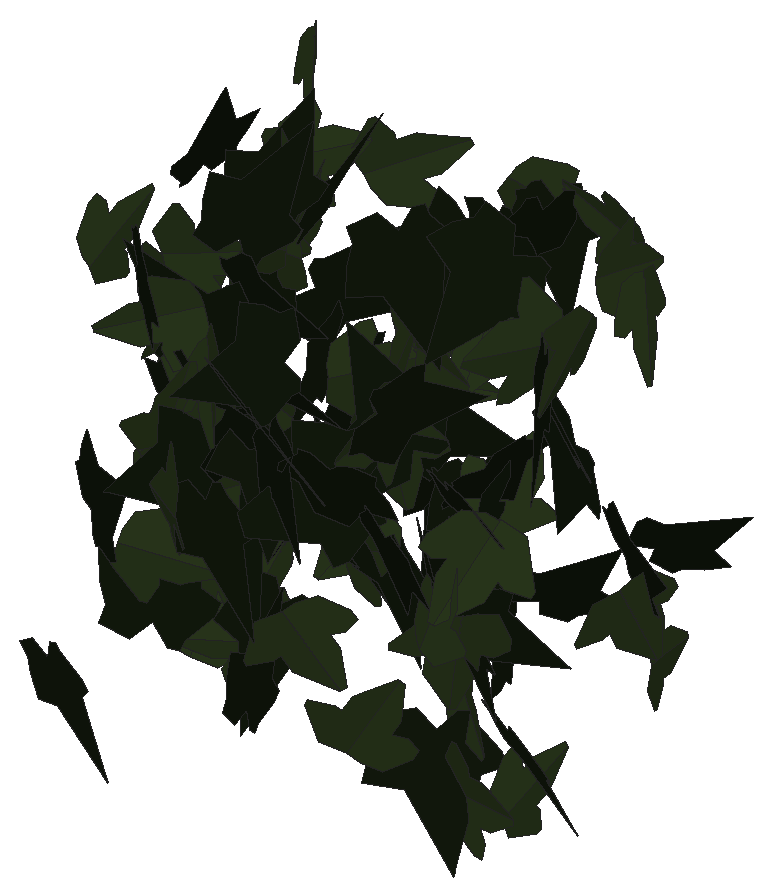
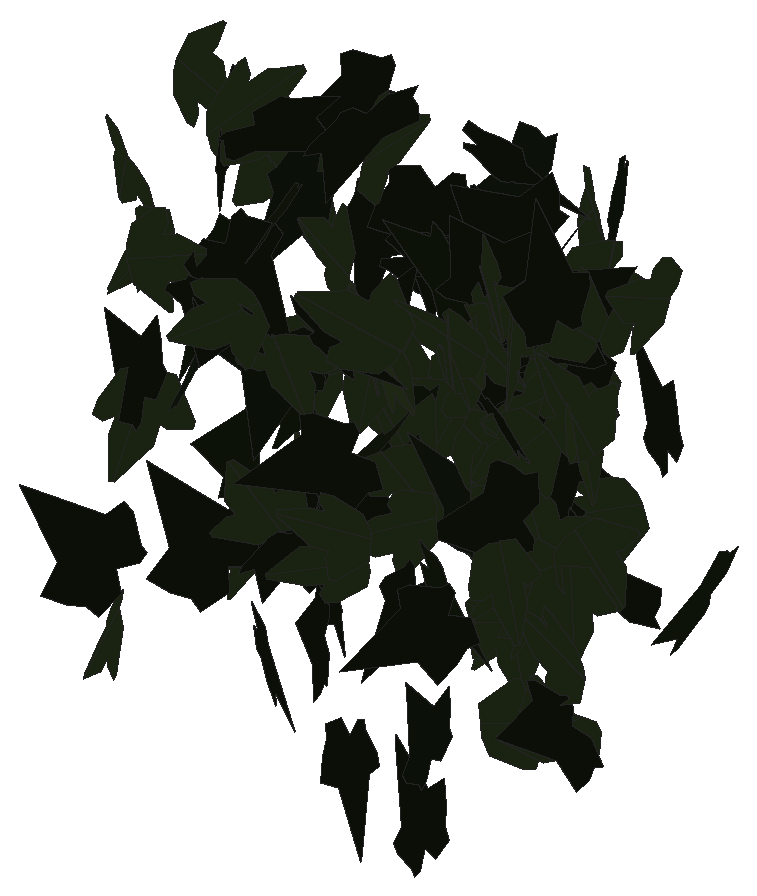
# SketchUp Ruby script. Lengths in inches.
U = 1.inch
M = Sketchup.active_model
def pt(a) = Geom::Point3d.new(a.map { |v| v * U })
def face(e, loops, mat)
  f = e.add_face(loops[0].map { |a| pt(a) })
  loops[1..].each { |l| e.add_face(l.map { |a| pt(a) }).erase! }
  f.material = f.back_material = mat if mat
  f
end
# faces: each face lists its corners as indices into pts; further lists are holes
def faces(e, pts, list, mat = nil) = list.each { |f| face(e, (f[0].is_a?(Array) ? f : [f]).map { |l| l.map { |i| pts[i] } }, mat) }
# xy, xz, yz: faces in a plane at the given z, y or x. An outline is a flat list of corners, or four numbers for a rectangle; further outlines are holes
def ring(l) = l.size == 4 ? [[l[0], l[1]], [l[2], l[1]], [l[2], l[3]], [l[0], l[3]]] : l.each_slice(2).to_a
def flat(e, list, mat, &to3) = list.each { |f| face(e, (f[0].is_a?(Array) ? f : [f]).map { |l| ring(l).map { |u, v| to3.(u, v) } }, mat) }
def xy(e, z, list, mat = nil) = flat(e, list, mat) { |x, y| [x, y, z] }
def xz(e, y, list, mat = nil) = flat(e, list, mat) { |x, z| [x, y, z] }
def yz(e, x, list, mat = nil) = flat(e, list, mat) { |y, z| [x, y, z] }
def lines(e, pts, list) = list.each { |a, b| e.add_line(pt(pts[a]), pt(pts[b])) }
# prism: a flat outline (further loops are holes) pulled along v
def prism(e, loops, v, mat = nil)
  f = face(e, loops, mat); d = Geom::Vector3d.new(v.map { |x| x * U })
  f.pushpull(f.normal.samedirection?(d) ? d.length : -d.length)
end
def box(e, o, s, mat = nil) = prism(e, [[o, [o[0] + s[0], o[1], o[2]], [o[0] + s[0], o[1] + s[1], o[2]], [o[0], o[1] + s[1], o[2]]]], [0, 0, s[2]], mat)
def at(x, y, z, deg = 0) = Geom::Transformation.translation(pt([x, y, z])) * Geom::Transformation.rotation(ORIGIN, Z_AXIS, deg.degrees)
def axes(o, x, y, z) = Geom::Transformation.new([*x, 0, *y, 0, *z, 0, *pt(o).to_a, 1])
def part(name) = M.definitions.add(name)
# library, detail: a bought-in or finely detailed component or shape, given as its bounding box
def library(name, o, s) = part(name).tap { |d| box(d.entities, o, s) }
def detail(e, o, s) = box(e.add_group.entities, o, s)
def put(e, d, t, mat = nil) = e.add_instance(d, t).tap { |i| i.material = mat if mat }
def group(e, t, mat = nil) = e.add_group.tap { |g| g.transformation = t; g.material = mat if mat }.entities
root = M.entities
M.materials.add("efeu1").color = [18, 25, 13]
M.materials.add("efeu2").color = [43, 57, 29]
c1 = part("ivyleaf_10")
p = [[0,0.5,-0.03],[-0.0625,2.02,-0.43],[-0.19,2.01,-0.46],[-0.54,1.05,-0.29],[-0.52,0.625,-0.18],[-0.83,0.76,-0.28],
  [-1.16,0.64,-0.33],[-1.15,0.33,-0.24],[-0.77,-0.39,0.02],[-0.3,-0.51,0.16],[0.04,-0.48,0.23],[-0.02,2.01,-0.4375],
  [-0.06,2.01,-0.43],[0.04,-0.49,0.23],[0.67,-0.49,0.14],[1.38,0.36,-0.2],[1.375,0.51,-0.24],[0.81,0.65,-0.19],
  [0.62,0.59,-0.15],[0.6,1.09,-0.28],[0.5,1.23,-0.31]]
faces(c1.entities,p,[[0,1,2,3,4,5,6,7,8,9,10],[11,12,0,13,14,15,16,17,18,19,20]],"efeu2")
c2 = part("ivyleaf_9")
p = [[1.54,2.16,1.25],[1.36,2.04,1.19],[-0.21,0.99,0.68],[-0.71,1.11,0.82],[-0.85,0.86,0.67],[-0.8,0.17,0.21],
  [-0.9,-0.01,0.1],[-0.67,-0.16,-0.02],[-0.08,-0.08,-0.05],[-0.03,-0.6,-0.4],[0.65,-0.88,-0.66],[0.83,-0.6,-0.49],
  [1.29,-0.42,-0.43],[1.8125,-0.07,-0.26],[1.21,0.44,0.15]]
faces(c2.entities,p,[[0,1,2,3,4,5,6,7,8,9,10,11,12,13,14]],"efeu1")
put(root,c1,axes([553.45,132.17,176.14],[-0.85734,-0.16884,0.1956],[-0.1875,-0.05992,-0.87353],[0.1778,-0.87732,0.02202]))
put(root,c1,axes([553.49,131.52,176.86],[-0.37338,-0.63209,0.40984],[-0.21331,-0.34998,-0.73412],[0.7225,-0.42999,-0.00494]))
put(root,c2,axes([553,137.13,177.71],[0.13734,0.14282,-0.8781],[-0.03731,0.88864,0.1387],[0.88885,0.01524,0.1415]))
put(root,c1,axes([553.22,129.19,182.25],[0.09536,0.36128,-0.85355],[0.25793,0.81382,0.37328],[0.89025,-0.27448,-0.01672]))
put(root,c2,axes([552.78,132.96,173.17],[0.0399,-0.18792,-0.90793],[0.81902,0.43308,-0.05365],[0.43457,-0.79897,0.18446]))
put(root,c1,axes([553.1,136.66,184.01],[0.52637,-0.38449,0.56942],[0.48204,-0.3045,-0.6512],[0.48961,0.71315,0.02895]))
put(root,c1,axes([552.74,133.1,174.82],[0.16897,-0.13445,-1.04144],[0.90074,-0.52365,0.21374],[-0.53977,-0.91594,0.03067]))
put(root,c1,axes([553.95,133.93,177.36],[-0.78131,0.01087,0.45029],[-0.45023,0.0071,-0.78139],[-0.01296,-0.90175,-0.00072]))
put(root,c1,axes([553.77,131.29,180.03],[0.19835,-0.98061,-0.08831],[-0.01984,0.08609,-1.00046],[0.98438,0.19933,-0.00237]))
put(root,c1,axes([553.29,131.76,179.94],[-0.70315,-0.10498,0.70648],[0.69807,0.10878,0.71094],[-0.15114,0.99081,-0.0032]))
put(root,c2,axes([553.57,132.45,183.16],[0.34971,0.64701,0.51065],[-0.25314,-0.4436,0.73541],[0.78442,-0.4316,0.00967]))
put(root,c2,axes([553.48,137.24,171.85],[-0.07363,-0.09714,0.93771],[0.45875,-0.82538,-0.04948],[0.82358,0.45107,0.1114]))
put(root,c2,axes([553.63,136.84,173.85],[0.12936,-0.34532,0.7892],[0.35441,-0.70605,-0.36703],[0.78516,0.37559,0.03565]))
put(root,c1,axes([553.95,131.74,171.8],[0.89509,0.30491,-0.29401],[0.26358,0.1371,0.94463],[0.33157,-0.93211,0.04277]))
put(root,c2,axes([554.6,135.55,177.55],[-0.80698,0.35413,-0.49466],[0.442,-0.22332,-0.88095],[-0.418,-0.9198,0.02344]))
put(root,c2,axes([553.91,126.625,173.33],[0.62055,-0.77596,0.01837],[0.01136,-0.01443,-0.99358],[0.7761,0.62065,-0.00014]))
put(root,c1,axes([554.59,132.6,182.65],[0.26858,-0.72193,-0.55385],[-0.08081,0.55627,-0.76426],[0.90631,0.26354,0.09599]))
put(root,c1,axes([554.28,131.86,176.05],[-0.6469,-0.18161,-0.77389],[0.75093,0.1877,-0.67175],[0.26077,-0.99104,0.0146]))
put(root,c1,axes([555.34,132.12,171.93],[0.02474,0.1004,0.93046],[-0.58665,-0.72354,0.09367],[0.72916,-0.58554,0.04379]))
put(root,c2,axes([554.13,133.08,178.01],[0.74933,-0.22892,0.45876],[0.43683,-0.14027,-0.7835],[0.26842,0.86734,-0.00563]))
put(root,c1,axes([554.48,132.22,179.54],[-0.67813,-0.01227,-0.5911],[0.59045,0.03186,-0.67806],[0.03018,-0.89902,-0.01596]))
put(root,c1,axes([554.27,130.71,181.79],[-0.30356,-0.12857,0.91473],[0.83448,0.37473,0.3296],[-0.39612,0.88796,-0.00665]))
put(root,c2,axes([555.28,137.625,173.97],[0.45363,0.06676,-0.79201],[-0.78602,-0.09761,-0.45843],[-0.11791,0.90749,0.00896]))
put(root,c2,axes([555.16,135.53,176.92],[-0.01441,0.02755,-0.86653],[-0.52306,0.69088,0.03067],[0.69141,0.52323,0.00514]))
put(root,c2,axes([555,128.875,173.89],[-0.89985,0.28307,0.57308],[0.53201,-0.21683,0.94246],[0.35428,1.04458,0.04033]))
put(root,c1,axes([554.94,131.17,176.19],[-0.71048,-0.38215,0.26134],[0.23759,0.1099,0.80659],[-0.39736,0.749,0.01499]))
put(root,c2,axes([555.1,132.95,180.58],[-0.73401,-0.01656,-0.54895],[0.54891,-0.05184,-0.73239],[-0.01781,-0.91511,0.05142]))
put(root,c2,axes([554.65,127.19,177.1875],[-0.0258,0.1064,0.9827],[0.40266,-0.89664,0.10765],[0.90271,0.403,-0.01994]))
put(root,c2,axes([555.16,131.15,178.37],[-0.63094,-0.62103,-0.26762],[0.17855,0.20004,-0.88515],[0.65224,-0.65551,-0.01658]))
put(root,c1,axes([555.74,128.88,181.71],[0.21403,0.12735,-0.91404],[-0.8221,-0.40005,-0.24824],[-0.41934,0.84926,0.02013]))
put(root,c1,axes([555.22,133.45,181.33],[0.27947,-0.67877,0.53629],[-0.20804,0.49431,0.73404],[-0.83967,-0.34839,-0.00337]))
put(root,c1,axes([555.1,131.05,174.49],[-0.03811,0.8763,0.22752],[-0.01095,0.22726,-0.87713],[-0.90529,-0.03964,0.00103]))
put(root,c1,axes([554.56,134.45,182.8],[0.37927,-0.1107,-0.83626],[0.84203,-0.00548,0.38261],[-0.05075,-0.91823,0.09854]))
put(root,c1,axes([555.96,132.4375,181.69],[-0.14778,0.02089,0.9241],[-0.92409,0.01827,-0.14819],[-0.02134,-0.93566,0.01774]))
put(root,c1,axes([555.24,131.17,179.73],[0.18415,0.16397,-0.89404],[0.16594,0.89081,0.19755],[0.89368,-0.19919,0.14754]))
put(root,c1,axes([555.49,131.67,174.45],[-0.50815,-0.73665,0.12773],[-0.0718,-0.10564,-0.89492],[0.74419,-0.5132,0.00088]))
put(root,c2,axes([555.78,127.36,183.52],[0.48196,-0.17025,-0.85565],[-0.80971,0.27662,-0.51113],[0.32479,0.94229,-0.00455]))
put(root,c1,axes([555.86,132.26,183.89],[0.60432,-0.60497,-0.52342],[-0.34245,0.39721,-0.85447],[0.72297,0.69383,0.03278]))
put(root,c2,axes([556.29,129.49,180.65],[0.20558,-0.112,1.07152],[-0.95634,0.48333,0.23401],[-0.49609,-0.97816,-0.00706]))
put(root,c1,axes([555.08,128.32,175.88],[-0.24512,-0.16136,-0.92547],[0.89167,0.26113,-0.28169],[0.29573,-0.92108,0.08227]))
put(root,c2,axes([555.69,132.08,183.11],[-0.44175,-0.25168,0.71456],[0.62093,0.35361,0.50842],[-0.43403,0.76204,0.00008]))
put(root,c1,axes([555.79,131.39,182.34],[-0.1845,-0.51425,-0.85622],[0.23069,0.82522,-0.54534],[0.97177,-0.29354,-0.0331]))
put(root,c1,axes([556.09,129.49,179.66],[-0.25113,-0.40608,0.90458],[-0.08561,-0.92078,-0.43712],[0.98785,-0.18303,0.19208]))
put(root,c1,axes([556,131.04,173.85],[0.19719,0.516,-0.72589],[0.21616,0.69351,0.5517],[0.86397,-0.29128,0.02765]))
put(root,c2,axes([555.91,129.17,178.24],[0.47202,0.56869,0.60064],[0.35877,0.48236,-0.73864],[-0.74529,0.59237,0.02484]))
put(root,c2,axes([556.16,129.21,177.99],[0.72515,0.61982,-0.03086],[-0.02463,-0.01867,-0.95395],[-0.6201,0.72556,0.00181]))
put(root,c1,axes([555.93,134.41,177.87],[0.017,-0.05018,-0.93059],[0.59762,0.71476,-0.02763],[0.71509,-0.59615,0.04521]))
put(root,c2,axes([556.23,130.38,183.17],[-0.28939,-0.1796,0.92444],[0.74911,0.54216,0.33984],[-0.57069,0.80274,-0.02269]))
put(root,c1,axes([556.35,127.71,179.46],[-0.44453,-0.82706,0.12784],[0.0608,0.11246,0.93895],[-0.83467,0.44867,0.00031]))
put(root,c1,axes([557.12,130.87,177.99],[-0.37275,-0.02316,0.83819],[-0.81883,-0.18747,-0.36932],[0.18057,-0.89797,0.05549]))
put(root,c2,axes([555.55,129.23,179.01],[0.35535,-0.23544,1.06071],[0.83933,-0.6492,-0.42528],[0.68997,0.911,-0.02894]))
put(root,c2,axes([556.13,129.84,176.51],[-0.47648,-0.33009,-0.79839],[0.64523,0.47036,-0.57954],[0.57452,-0.80201,-0.01129]))
put(root,c1,axes([556.8,130.83,177.15],[0.02787,-0.00437,-0.91531],[-0.4805,-0.77948,-0.01091],[-0.77906,0.48061,-0.02601]))
put(root,c2,axes([556.58,132.24,182.77],[-0.32957,0.92555,0.04367],[0.01391,-0.0414,0.98248],[0.92648,0.32987,0.00078]))
put(root,c2,axes([557.09,127.72,178.84],[-0.30302,-0.32577,0.79941],[-0.43706,-0.67272,-0.43982],[0.74442,-0.52757,0.06719]))
put(root,c1,axes([556.41,135.14,182.74],[-0.36565,-0.34592,0.89352],[0.66527,0.5966,0.50321],[-0.68953,0.75905,0.01168]))
put(root,c1,axes([556.29,136.36,178.32],[0.00967,-0.03559,-0.88536],[0.8859,-0.01726,0.01037],[-0.01766,-0.88524,0.0354]))
put(root,c2,axes([556.34,130.22,181.83],[0.57175,0.01164,-0.82271],[0.78741,0.28289,0.55122],[0.23869,-0.9611,0.15229]))
put(root,c1,axes([556.72,135.91,177.25],[0.09076,0.07216,0.87669],[0.55294,0.68078,-0.11328],[-0.68414,0.55979,0.02476]))
put(root,c2,axes([557.3,130.68,175.9375],[-0.07689,0.89712,0.18789],[0.00301,-0.1883,0.90031],[0.91657,0.07587,0.01281]))
put(root,c1,axes([557,128.08,181.33],[0.54752,-0.25034,0.82787],[0.72731,-0.39694,-0.60105],[0.46803,0.90971,-0.03444]))
put(root,c2,axes([557.8,129.72,174.67],[-0.84819,-0.26055,-0.44335],[0.42219,0.13541,-0.88729],[0.2936,-0.94744,-0.00489]))
put(root,c2,axes([558.82,134.3125,181.66],[-0.56284,0.31778,0.65359],[-0.56567,0.32745,-0.64633],[-0.45627,-0.79796,-0.00494]))
put(root,c2,axes([558,129.32,179.08],[-0.55819,-0.56935,-0.43165],[0.29491,0.31533,-0.79728],[0.65078,-0.63124,-0.00895]))
put(root,c2,axes([558.5625,127.67,173.45],[-0.10909,-0.2453,0.88445],[0.34212,0.81562,0.26841],[-0.8517,0.35905,-0.00547]))
put(root,c1,axes([559.45,124.01,180.21],[-0.14653,0.10602,0.99224],[-0.90624,0.40571,-0.17718],[-0.41776,-0.91729,0.03632]))
put(root,c1,axes([559.21,131.05,176.72],[0.77221,0.09324,-0.50297],[-0.50228,-0.03437,-0.77751],[-0.09693,0.92093,0.02191]))
put(root,c1,axes([559.18,131.38,179.66],[0.33999,-0.76959,0.3817],[0.15784,-0.34756,-0.84134],[0.84443,0.37482,0.00357]))
put(root,c1,axes([559.43,132.13,181.15],[0.59071,-0.69928,-0.33576],[-0.21209,0.26036,-0.91537],[0.74615,0.62761,0.00563]))
put(root,c2,axes([559.97,127,182.75],[-0.8753,0.1588,0.38799],[-0.3814,0.07123,-0.88958],[-0.17404,-0.95478,-0.00184]))
put(root,c2,axes([558.92,133.85,175.31],[-0.40072,0.0543,-0.94422],[0.93949,-0.09517,-0.40418],[-0.10885,-1.0213,-0.01253]))
put(root,c2,axes([558.8125,133.33,178.14],[0.17029,0.13493,-0.8697],[0.34335,0.80545,0.19219],[0.81036,-0.36962,0.10133]))
put(root,c2,axes([559.19,125.48,179.56],[0.4821,-0.94802,-0.08604],[-0.03933,0.07652,-1.06356],[0.95111,0.4837,-0.00037]))
put(root,c2,axes([558.99,126.66,181.85],[0.84856,-0.64268,0.34444],[0.28298,-0.19681,-1.06439],[0.67201,0.89441,0.01329]))
put(root,c2,axes([559.48,134.47,176.35],[0.09216,-0.86475,-0.31916],[-0.03374,0.31737,-0.86965],[0.92115,0.09814,0.00008]))
put(root,c1,axes([559.47,136.33,182.89],[-0.5043,-0.06075,-0.75277],[0.74428,0.11352,-0.50778],[0.12807,-0.89895,-0.01325]))
put(root,c2,axes([559.39,133.43,173.37],[0.12479,-0.07977,-0.92172],[0.91577,-0.12157,0.1345],[-0.13153,-0.92215,0.062]))
put(root,c2,axes([560.65,134.1,173.2],[-0.18263,0.04433,-0.93711],[-0.932,0.10065,0.1864],[0.10733,0.94942,0.02399]))
put(root,c1,axes([560.07,134.0625,180.7],[0.87905,0.22774,-0.19223],[-0.19173,-0.02621,-0.9078],[-0.22816,0.89944,0.02222]))
put(root,c1,axes([560.14,130.68,179.36],[-0.83444,-0.58537,-0.12744],[0.10366,0.07413,-1.01929],[0.59004,-0.84085,-0.00115]))
put(root,c2,axes([559.56,129.95,176.98],[0.67339,-0.59575,0.122],[0.09659,-0.07494,-0.89907],[0.6004,0.68024,0.00781]))
put(root,c1,axes([559.5,130.09,176.49],[-0.50506,-0.02168,0.90204],[0.89902,-0.10013,0.50096],[0.07685,1.02895,0.06776]))
put(root,c2,axes([560.58,130.78,179.26],[-0.62123,-0.80256,0.2106],[0.14684,0.15259,1.01465],[-0.81663,0.63796,0.02225]))
put(root,c2,axes([559.73,127.01,180.67],[-0.20309,-0.0196,-0.94676],[0.94657,0.02388,-0.20354],[0.02746,-0.968,0.01415]))
put(root,c2,axes([560.3125,136.2,182.78],[-0.53484,-0.33666,-0.65792],[0.5731,0.32386,-0.63161],[0.46664,-0.78361,0.02162]))
put(root,c2,axes([560.09,130.58,176.6],[0.38435,-0.89886,0.23349],[0.1228,-0.20129,-0.97703],[0.92053,0.40216,0.03285]))
put(root,c1,axes([560.47,126.9,176.45],[-0.71224,-0.58375,-0.47634],[0.40083,0.26145,-0.91974],[0.63796,-0.81599,0.04607]))
put(root,c2,axes([561.44,127.75,179.78],[-0.96645,-0.13213,0.57145],[-0.56613,-0.0778,-0.97544],[0.15333,-1.12005,0.00034]))
put(root,c1,axes([560.375,134.03,176.24],[0.67499,0.44572,-0.49084],[0.41268,0.26579,0.80886],[0.51893,-0.79113,-0.00479]))
put(root,c2,axes([560.93,134.88,183.32],[-0.2624,0.64473,-0.79081],[0.29747,-0.73273,-0.69608],[-0.976,-0.39666,0.00046]))
put(root,c2,axes([560.71,130.27,184.74],[0.08424,-0.92547,-0.48982],[-0.05041,0.48724,-0.92928],[1.04589,0.09803,-0.00534]))
put(root,c2,axes([560.63,133.79,183.48],[0.42887,-0.84097,0.0972],[0.04511,-0.0861,-0.94402],[0.84537,0.43124,0.00106]))
put(root,c2,axes([561.62,130.71,174.76],[0.05464,-0.51843,0.78811],[-0.1254,0.77843,0.52076],[-0.93497,-0.13471,-0.02379]))
put(root,c1,axes([560.72,131.11,181.35],[-0.15325,-0.01332,0.92108],[0.91078,-0.1421,0.14948],[0.13803,0.92287,0.03631]))
put(root,c2,axes([561.73,126.59,180.81],[0.63218,0.47432,-0.58118],[-0.49473,-0.30772,-0.78927],[-0.56391,0.80171,0.0409]))
put(root,c2,axes([561.28,131.5625,174.82],[0.04384,0.08836,-0.92981],[0.37698,0.84997,0.09855],[0.85454,-0.37949,0.00423]))
put(root,c1,axes([562.56,135.78,182.96],[-0.30339,0.1796,-0.85444],[-0.82798,0.22789,0.3419],[0.2771,0.8776,0.08607]))
put(root,c2,axes([562.26,131.36,179],[0.21794,0.94679,0.11276],[0.02045,0.111,-0.97154],[-0.95326,0.21884,0.00494]))
put(root,c2,axes([561.89,133.82,174.55],[0.74663,0.59788,-0.11369],[0.07963,0.08243,0.9564],[0.60336,-0.75072,0.01447]))
put(root,c1,axes([562.59,127.67,182.02],[-0.00517,0.11546,-1.04342],[-0.16214,-1.031,-0.11329],[-1.03719,0.1606,0.02291]))
put(root,c2,axes([562.76,131.52,184.35],[-0.61523,-0.78409,0.31422],[-0.19628,-0.24539,-0.99665],[0.82159,-0.64578,-0.0028]))
put(root,c2,axes([562.9,130.9,178.52],[-0.74515,0.47072,-0.34018],[0.29176,-0.17508,-0.88135],[-0.50217,-0.8002,-0.00727]))
put(root,c1,axes([563.1,134.69,182.65],[-0.05087,0.15909,0.89723],[-0.2315,0.86688,-0.16683],[-0.88132,-0.23689,-0.00797]))
put(root,c1,axes([562.85,126.13,174.71],[-0.80085,-0.49624,0.46193],[0.40441,0.22415,0.94192],[-0.54414,0.89694,0.02018]))
put(root,c2,axes([562.92,128.8,173.7],[-0.41463,-0.79078,-0.5533],[0.25506,0.49101,-0.89289],[0.93082,-0.48679,-0.0018]))
put(root,c2,axes([563.375,126.47,179.74],[0.71709,0.05236,-0.68362],[-0.68421,-0.00897,-0.71839],[-0.04409,0.9907,0.02963]))
put(root,c2,axes([563.21,126.53,182.83],[0.03191,0.40173,-0.86173],[-0.13753,0.85509,0.39354],[0.94077,0.11138,0.08676]))
put(root,c2,axes([563.37,131.91,181.03],[0.82171,-0.16314,-0.62354],[-0.60323,0.16117,-0.83712],[0.227,1.01884,0.03258]))
put(root,c2,axes([563.03,133.43,178.9],[0.10128,-0.72727,0.75792],[0.07572,-0.7544,-0.73401],[1.04768,0.12483,-0.02022]))
put(root,c1,axes([562.88,129.65,174.35],[0.27573,-0.08015,0.86159],[0.80258,-0.31435,-0.28608],[0.32347,0.84826,-0.02461]))
put(root,c1,axes([563.74,135.37,173.04],[0.13574,-0.20911,-0.8898],[-0.05583,0.89598,-0.21909],[0.91234,0.08595,0.11898]))
put(root,c2,axes([563.07,129.38,176.34],[0.4186,-0.72926,0.48341],[0.22947,-0.42562,-0.84079],[0.8443,0.47724,-0.01115]))
put(root,c2,axes([563.09,136.33,175.14],[0.67658,0.5524,-0.30883],[0.2415,0.19253,0.87344],[0.58498,-0.71838,-0.00339]))
put(root,c1,axes([564.06,128.16,176.97],[-0.69289,-0.8151,0.09386],[-0.05808,-0.07381,-1.0698],[0.81843,-0.69531,0.00354]))
put(root,c1,axes([563.67,128.69,172.46],[-0.27447,-0.00104,1.01632],[1.01049,-0.11287,0.27278],[0.1087,1.04666,0.03043]))
put(root,c1,axes([564.47,130.375,183.29],[-0.03034,0.29409,1.10951],[0.12736,-1.10218,0.29563],[1.14074,0.13088,-0.0035]))
put(root,c1,axes([564.45,129.54,172.23],[0.10231,0.30324,-0.85805],[0.24896,0.8212,0.31989],[0.87534,-0.269,0.00931]))
put(root,c2,axes([564.39,127.53,180.74],[0.98261,-0.09894,-0.30044],[-0.29773,0.04177,-0.98751],[0.10681,1.02666,0.01122]))
put(root,c1,axes([564.64,126.43,177.98],[0.82269,-0.43799,-0.23201],[0.20996,-0.09929,0.93195],[-0.44898,-0.84899,0.0107]))
put(root,c2,axes([564.89,130.07,183.04],[-0.1724,0.11665,-1.07675],[0.97821,-0.4512,-0.2055],[-0.46485,-0.99274,-0.03312]))
put(root,c1,axes([564.95,133.37,183.43],[0.73282,-0.25754,0.60784],[0.56544,-0.22381,-0.77653],[0.34069,0.92542,-0.01865]))
put(root,c1,axes([565.7,127.03,180.28],[0.8026,0.49068,-0.51447],[-0.4405,-0.2658,-0.94071],[-0.55804,0.91553,0.00262]))
put(root,c2,axes([564.93,128.9,174.36],[0.60465,-0.65906,0.42677],[0.30314,-0.30094,-0.89423],[0.7243,0.67615,0.01798]))
put(root,c1,axes([565.73,131.88,176.69],[-0.44472,-0.82261,-0.42579],[0.21458,0.36799,-0.93504],[0.90108,-0.49363,0.01251]))
put(root,c2,axes([565.13,132.68,177.22],[0.16693,-0.27808,0.91196],[0.45946,-0.78777,-0.32431],[0.8354,0.48883,-0.00386]))
put(root,c1,axes([565.79,130.15,184.13],[0.1304,-0.68343,0.67365],[0.19437,-0.64694,-0.69396],[0.93974,0.22864,0.05006]))
